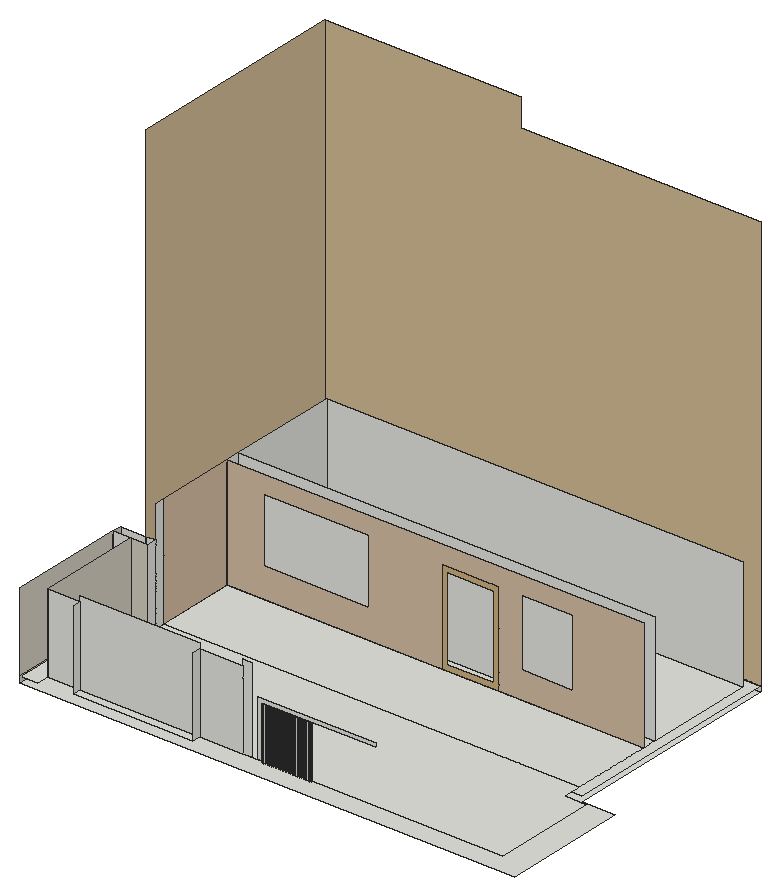
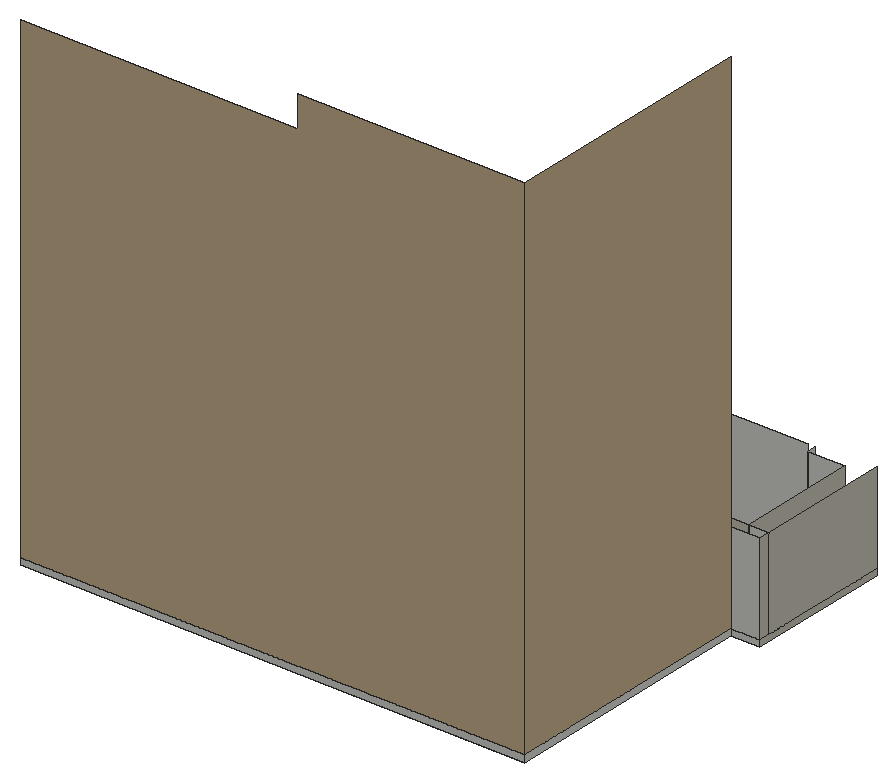
# SketchUp Ruby script. Lengths in inches.
U = 1.inch
M = Sketchup.active_model
def pt(a) = Geom::Point3d.new(a.map { |v| v * U })
def face(e, loops, mat)
  f = e.add_face(loops[0].map { |a| pt(a) })
  loops[1..].each { |l| e.add_face(l.map { |a| pt(a) }).erase! }
  f.material = f.back_material = mat if mat
  f
end
# faces: each face lists its corners as indices into pts; further lists are holes
def faces(e, pts, list, mat = nil) = list.each { |f| face(e, (f[0].is_a?(Array) ? f : [f]).map { |l| l.map { |i| pts[i] } }, mat) }
# xy, xz, yz: faces in a plane at the given z, y or x. An outline is a flat list of corners, or four numbers for a rectangle; further outlines are holes
def ring(l) = l.size == 4 ? [[l[0], l[1]], [l[2], l[1]], [l[2], l[3]], [l[0], l[3]]] : l.each_slice(2).to_a
def flat(e, list, mat, &to3) = list.each { |f| face(e, (f[0].is_a?(Array) ? f : [f]).map { |l| ring(l).map { |u, v| to3.(u, v) } }, mat) }
def xy(e, z, list, mat = nil) = flat(e, list, mat) { |x, y| [x, y, z] }
def xz(e, y, list, mat = nil) = flat(e, list, mat) { |x, z| [x, y, z] }
def yz(e, x, list, mat = nil) = flat(e, list, mat) { |y, z| [x, y, z] }
def lines(e, pts, list) = list.each { |a, b| e.add_line(pt(pts[a]), pt(pts[b])) }
# prism: a flat outline (further loops are holes) pulled along v
def prism(e, loops, v, mat = nil)
  f = face(e, loops, mat); d = Geom::Vector3d.new(v.map { |x| x * U })
  f.pushpull(f.normal.samedirection?(d) ? d.length : -d.length)
end
def box(e, o, s, mat = nil) = prism(e, [[o, [o[0] + s[0], o[1], o[2]], [o[0] + s[0], o[1] + s[1], o[2]], [o[0], o[1] + s[1], o[2]]]], [0, 0, s[2]], mat)
def at(x, y, z, deg = 0) = Geom::Transformation.translation(pt([x, y, z])) * Geom::Transformation.rotation(ORIGIN, Z_AXIS, deg.degrees)
def axes(o, x, y, z) = Geom::Transformation.new([*x, 0, *y, 0, *z, 0, *pt(o).to_a, 1])
def part(name) = M.definitions.add(name)
# library, detail: a bought-in or finely detailed component or shape, given as its bounding box
def library(name, o, s) = part(name).tap { |d| box(d.entities, o, s) }
def detail(e, o, s) = box(e.add_group.entities, o, s)
def put(e, d, t, mat = nil) = e.add_instance(d, t).tap { |i| i.material = mat if mat }
def group(e, t, mat = nil) = e.add_group.tap { |g| g.transformation = t; g.material = mat if mat }.entities
root = M.entities
M.materials.add("[Formica Beige]").color = [211, 187, 149]
M.materials.add("[Formica Graystone]").color = [209, 204, 189]
M.materials.add("[Formica Laminate Light]").color = [213, 189, 164]
M.materials.add("[Wood Floor Light]").color = [204, 176, 127]
xy(root,0,[[0,1.67,0,203.79,40.4375,203.79,40.4375,563.79,742.93,563.79,742.93,203.79,797.12,203.79,797.12,1.67]])
xy(root,9,[[0,1.67,28.1,189.01],[80.35,8.25,273.1875,21.38],[28.1,21.38,762.14,21.38,762.14,189.01,727.17,189.01,727.17,219.56,56.2,219.56,56.2,189.01,28.1,189.01],[0,189.01,56.2,203.79],[40.4375,203.79,40.4375,563.79,742.93,563.79,742.93,203.79,727.17,203.79,727.17,548.03,56.2,548.03,56.2,203.79],
  [56.2,219.56,727.17,348.07],[56.2,348.07,727.17,370.07],[56.2,370.07,727.17,548.03]])
xz(root,17.41,[[370.65,12.5,370.65,102.25,560.77,102.25,560.77,96.37,377.34,96.37,377.34,12.5]])
xz(root,21.38,[[28.1,9,80.35,136.125],[80.35,9,273.1875,145.125],[273.1875,9,342.51,136.125],[342.51,9,357.9375,145.125]])
xz(root,189.01,[[0,9,28.1,136.125]])
xz(root,189.01,[[28.1,9,56.2,136.125]],"[Formica Graystone]")
xz(root,203.79,[[0,0,40.4375,9],[0,9,40.4375,136.125],[40.4375,9,56.2,136.125]])
xz(root,348.07,[[[56.2,9,401.38,9,401.38,160.08,494.76,160.08,494.76,9,727.17,9,727.17,189,56.2,189],[116.08,56.31,284.86,160.63],[530.86,51.82,613.92,160.38]]],"[Formica Laminate Light]")
xz(root,348.07,[[[401.38,9,494.76,160.08],[410.04,17.66,486.1,151.43]]],"[Wood Floor Light]")
xz(root,370.07,[[56.2,9,727.17,189]])
xz(root,548.03,[[56.2,9,727.17,189]])
xz(root,563.79,[[40.4375,0,742.93,9]])
xz(root,563.79,[[40.4375,9,40.4375,723.1875,356.6875,723.1875,356.6875,679.64,742.93,679.64,742.93,9]],"[Formica Beige]")
yz(root,0,[[1.67,0,203.79,9],[1.67,9,189.01,136.125],[189.01,9,203.79,136.125]],"[Formica Graystone]")
yz(root,28.1,[[21.38,9,189.01,136.125]],"[Formica Graystone]")
yz(root,40.4375,[[203.79,0,563.79,9]])
yz(root,40.4375,[[203.79,9,563.79,723.1875]],"[Formica Beige]")
yz(root,56.2,[[189.01,9,203.79,136.125],[203.79,9,219.56,189],[348.07,9,370.07,189],[370.07,9,548.03,189]])
yz(root,56.2,[[219.56,9,348.07,189]],"[Formica Laminate Light]")
yz(root,80.35,[[8.25,9,21.38,136.125]])
yz(root,273.1875,[[8.25,9,21.38,136.125]])
p = [[381.39,13.76,12.5],[381.35,14.08,12.5],[381.35,14.08,96.37],[381.39,13.76,96.37],[383.49,14.08,12.5],[383.45,13.76,12.5],
  [383.45,13.76,96.37],[383.49,14.08,96.37],[385.95,13.76,12.5],[385.91,14.08,12.5],[385.91,14.08,96.37],[385.95,13.76,96.37],
  [389.24,14.08,12.5],[389.2,13.76,12.5],[389.2,13.76,96.37],[389.24,14.08,96.37],[391.7,13.76,12.5],[391.66,14.08,12.5],
  [391.66,14.08,96.37],[391.7,13.76,96.37],[395.74,14.08,12.5],[395.7,13.76,12.5],[395.7,13.76,96.37],[395.74,14.08,96.37],
  [398.2,13.76,12.5],[398.16,14.08,12.5],[398.16,14.08,96.37],[398.2,13.76,96.37],[401.37,14.08,12.5],[401.33,13.76,12.5],
  [401.33,13.76,96.37],[401.37,14.08,96.37],[403.83,13.76,12.5],[403.78,14.08,12.5],[403.78,14.08,96.37],[403.83,13.76,96.37],
  [407.24,14.08,12.5],[407.2,13.76,12.5],[407.2,13.76,96.37],[407.24,14.08,96.37],[409.7,13.76,12.5],[409.66,14.08,12.5],
  [409.66,14.08,96.37],[409.7,13.76,96.37],[412.81,14.08,12.5],[412.76,13.76,12.5],[412.76,13.76,96.37],[412.81,14.08,96.37],
  [415.26,13.76,12.5],[415.22,14.08,12.5],[415.22,14.08,96.37],[415.26,13.76,96.37],[417.68,14.08,12.5],[417.64,13.76,12.5],
  [417.64,13.76,96.37],[417.68,14.08,96.37],[420.14,13.76,12.5],[420.1,14.08,12.5],[420.1,14.08,96.37],[420.14,13.76,96.37],
  [423.43,14.08,12.5],[423.39,13.76,12.5],[423.39,13.76,96.37],[423.43,14.08,96.37],[425.89,13.76,12.5],[425.85,14.08,12.5],
  [425.85,14.08,96.37],[425.89,13.76,96.37],[429.31,14.08,12.5],[429.26,13.76,12.5],[429.26,13.76,96.37],[429.31,14.08,96.37],
  [431.76,13.76,12.5],[431.72,14.08,12.5],[431.72,14.08,96.37],[431.76,13.76,96.37],[434.99,14.08,12.5],[434.95,13.76,12.5],
  [434.95,13.76,96.37],[434.99,14.08,96.37],[437.45,13.76,12.5],[437.41,14.08,12.5],[437.41,14.08,96.37],[437.45,13.76,96.37],
  [441.24,14.08,12.5],[441.2,13.76,12.5],[441.2,13.76,96.37],[441.24,14.08,96.37],[443.7,13.76,12.5],[443.66,14.08,12.5],
  [443.66,14.08,96.37],[443.7,13.76,96.37],[447.24,14.08,12.5],[447.2,13.76,12.5],[447.2,13.76,96.37],[447.24,14.08,96.37],
  [449.7,13.76,12.5],[449.66,14.08,12.5],[449.66,14.08,96.37],[449.7,13.76,96.37],[452.74,14.08,12.5],[452.7,13.76,12.5],
  [452.7,13.76,96.37],[452.74,14.08,96.37],[455.2,13.76,12.5],[455.16,14.08,12.5],[455.16,14.08,96.37],[455.2,13.76,96.37],
  [457.43,14.08,12.5],[457.39,13.76,12.5],[457.39,13.76,96.37],[457.43,14.08,96.37],[379.06,14.38,12.5],[378.94,14.08,12.5],
  [378.94,14.08,96.37],[379.06,14.38,96.37],[381.23,14.38,12.5],[381.23,14.38,96.37],[383.62,14.38,12.5],[383.62,14.38,96.37],
  [385.78,14.38,12.5],[385.78,14.38,96.37],[389.37,14.38,12.5],[389.37,14.38,96.37],[391.53,14.38,12.5],[391.53,14.38,96.37],
  [395.87,14.38,12.5],[395.87,14.38,96.37],[398.03,14.38,12.5],[398.03,14.38,96.37],[401.49,14.38,12.5],[401.49,14.38,96.37],
  [403.66,14.38,12.5],[403.66,14.38,96.37],[407.37,14.38,12.5],[407.37,14.38,96.37],[409.53,14.38,12.5],[409.53,14.38,96.37],
  [412.93,14.38,12.5],[412.93,14.38,96.37],[415.1,14.38,12.5],[415.1,14.38,96.37],[417.81,14.38,12.5],[417.81,14.38,96.37],
  [419.97,14.38,12.5],[419.97,14.38,96.37],[423.56,14.38,12.5],[423.56,14.38,96.37],[425.72,14.38,12.5],[425.72,14.38,96.37],
  [429.43,14.38,12.5],[429.43,14.38,96.37],[431.6,14.38,12.5],[431.6,14.38,96.37],[435.12,14.38,12.5],[435.12,14.38,96.37],
  [437.28,14.38,12.5],[437.28,14.38,96.37],[441.37,14.38,12.5],[441.37,14.38,96.37],[443.53,14.38,12.5],[443.53,14.38,96.37],
  [447.37,14.38,12.5],[447.37,14.38,96.37],[449.53,14.38,12.5],[449.53,14.38,96.37],[452.87,14.38,12.5],[452.87,14.38,96.37],
  [455.03,14.38,12.5],[455.03,14.38,96.37],[457.56,14.38,12.5],[457.56,14.38,96.37],[379.26,14.64,12.5],[379.26,14.64,96.37],
  [381.03,14.64,12.5],[381.03,14.64,96.37],[383.82,14.64,12.5],[383.82,14.64,96.37],[385.59,14.64,12.5],[385.59,14.64,96.37],
  [389.57,14.64,12.5],[389.57,14.64,96.37],[391.34,14.64,12.5],[391.34,14.64,96.37],[396.07,14.64,12.5],[396.07,14.64,96.37],
  [397.84,14.64,12.5],[397.84,14.64,96.37],[401.69,14.64,12.5],[401.69,14.64,96.37],[403.46,14.64,12.5],[403.46,14.64,96.37],
  [407.57,14.64,12.5],[407.57,14.64,96.37],[409.34,14.64,12.5],[409.34,14.64,96.37],[413.13,14.64,12.5],[413.13,14.64,96.37],
  [414.9,14.64,12.5],[414.9,14.64,96.37],[418.01,14.64,12.5],[418.01,14.64,96.37],[419.77,14.64,12.5],[419.77,14.64,96.37],
  [423.76,14.64,12.5],[423.76,14.64,96.37],[425.52,14.64,12.5],[425.52,14.64,96.37],[429.63,14.64,12.5],[429.63,14.64,96.37],
  [431.4,14.64,12.5],[431.4,14.64,96.37],[435.32,14.64,12.5],[435.32,14.64,96.37],[437.09,14.64,12.5],[437.09,14.64,96.37],
  [441.57,14.64,12.5],[441.57,14.64,96.37],[443.34,14.64,12.5],[443.34,14.64,96.37],[447.57,14.64,12.5],[447.57,14.64,96.37],
  [449.34,14.64,12.5],[449.34,14.64,96.37],[453.07,14.64,12.5],[453.07,14.64,96.37],[454.84,14.64,12.5],[454.84,14.64,96.37],
  [457.76,14.64,12.5],[457.76,14.64,96.37],[459.72,14.38,12.5],[459.52,14.64,12.5],[459.52,14.64,96.37],[459.72,14.38,96.37],
  [379.52,14.84,12.5],[379.52,14.84,96.37],[380.77,14.84,12.5],[380.77,14.84,96.37],[384.08,14.84,12.5],[384.08,14.84,96.37],
  [385.33,14.84,12.5],[385.33,14.84,96.37],[389.83,14.84,12.5],[389.83,14.84,96.37],[391.08,14.84,12.5],[391.08,14.84,96.37],
  [396.33,14.84,12.5],[396.33,14.84,96.37],[397.58,14.84,12.5],[397.58,14.84,96.37],[401.95,14.84,12.5],[401.95,14.84,96.37],
  [403.2,14.84,12.5],[403.2,14.84,96.37],[407.83,14.84,12.5],[407.83,14.84,96.37],[409.08,14.84,12.5],[409.08,14.84,96.37],
  [413.39,14.84,12.5],[413.39,14.84,96.37],[414.64,14.84,12.5],[414.64,14.84,96.37],[418.26,14.84,12.5],[418.26,14.84,96.37],
  [419.51,14.84,12.5],[419.51,14.84,96.37],[424.01,14.84,12.5],[424.01,14.84,96.37],[425.26,14.84,12.5],[425.26,14.84,96.37],
  [429.89,14.84,12.5],[429.89,14.84,96.37],[431.14,14.84,12.5],[431.14,14.84,96.37],[435.58,14.84,12.5],[435.58,14.84,96.37],
  [436.83,14.84,12.5],[436.83,14.84,96.37],[441.83,14.84,12.5],[441.83,14.84,96.37],[443.08,14.84,12.5],[443.08,14.84,96.37],
  [447.83,14.84,12.5],[447.83,14.84,96.37],[449.08,14.84,12.5],[449.08,14.84,96.37],[453.33,14.84,12.5],[453.33,14.84,96.37],
  [454.58,14.84,12.5],[454.58,14.84,96.37],[458.01,14.84,12.5],[458.01,14.84,96.37],[459.26,14.84,12.5],[459.26,14.84,96.37],
  [379.82,14.96,12.5],[379.82,14.96,96.37],[380.47,14.96,12.5],[380.47,14.96,96.37],[384.38,14.96,12.5],[384.38,14.96,96.37],
  [385.03,14.96,12.5],[385.03,14.96,96.37],[390.13,14.96,12.5],[390.13,14.96,96.37],[390.78,14.96,12.5],[390.78,14.96,96.37],
  [396.63,14.96,12.5],[396.63,14.96,96.37],[397.28,14.96,12.5],[397.28,14.96,96.37],[402.25,14.96,12.5],[402.25,14.96,96.37],
  [402.9,14.96,12.5],[402.9,14.96,96.37],[408.13,14.96,12.5],[408.13,14.96,96.37],[408.78,14.96,12.5],[408.78,14.96,96.37],
  [413.69,14.96,12.5],[413.69,14.96,96.37],[414.34,14.96,12.5],[414.34,14.96,96.37],[418.57,14.96,12.5],[418.57,14.96,96.37],
  [419.21,14.96,12.5],[419.21,14.96,96.37],[424.32,14.96,12.5],[424.32,14.96,96.37],[424.96,14.96,12.5],[424.96,14.96,96.37],
  [430.19,14.96,12.5],[430.19,14.96,96.37],[430.84,14.96,12.5],[430.84,14.96,96.37],[435.88,14.96,12.5],[435.88,14.96,96.37],
  [436.53,14.96,12.5],[436.53,14.96,96.37],[442.13,14.96,12.5],[442.13,14.96,96.37],[442.78,14.96,12.5],[442.78,14.96,96.37],
  [448.13,14.96,12.5],[448.13,14.96,96.37],[448.78,14.96,12.5],[448.78,14.96,96.37],[453.63,14.96,12.5],[453.63,14.96,96.37],
  [454.28,14.96,12.5],[454.28,14.96,96.37],[458.32,14.96,12.5],[458.32,14.96,96.37],[458.96,14.96,12.5],[458.96,14.96,96.37],
  [380.14,15.01,12.5],[380.14,15.01,96.37],[384.7,15.01,12.5],[384.7,15.01,96.37],[390.45,15.01,12.5],[390.45,15.01,96.37],
  [396.95,15.01,12.5],[396.95,15.01,96.37],[402.58,15.01,12.5],[402.58,15.01,96.37],[408.45,15.01,12.5],[408.45,15.01,96.37],
  [414.01,15.01,12.5],[414.01,15.01,96.37],[418.89,15.01,12.5],[418.89,15.01,96.37],[424.64,15.01,12.5],[424.64,15.01,96.37],
  [430.51,15.01,12.5],[430.51,15.01,96.37],[436.2,15.01,12.5],[436.2,15.01,96.37],[442.45,15.01,12.5],[442.45,15.01,96.37],
  [448.45,15.01,12.5],[448.45,15.01,96.37],[453.95,15.01,12.5],[453.95,15.01,96.37],[458.64,15.01,12.5],[458.64,15.01,96.37]]
faces(root,p,[[0,1,2,3],[4,5,6,7],[8,9,10,11],[12,13,14,15],[16,17,18,19],[20,21,22,23],[24,25,26,27],[28,29,30,31],
  [32,33,34,35],[36,37,38,39],[40,41,42,43],[44,45,46,47],[48,49,50,51],[52,53,54,55],[56,57,58,59],[60,61,62,63],
  [64,65,66,67],[68,69,70,71],[72,73,74,75],[76,77,78,79],[80,81,82,83],[84,85,86,87],[88,89,90,91],[92,93,94,95],
  [96,97,98,99],[100,101,102,103],[104,105,106,107],[108,109,110,111],[112,113,114,115],[1,116,117,2],[118,4,7,119],[9,120,121,10],
  [122,12,15,123],[17,124,125,18],[126,20,23,127],[25,128,129,26],[130,28,31,131],[33,132,133,34],[134,36,39,135],[41,136,137,42],
  [138,44,47,139],[49,140,141,50],[142,52,55,143],[57,144,145,58],[146,60,63,147],[65,148,149,66],[150,68,71,151],[73,152,153,74],
  [154,76,79,155],[81,156,157,82],[158,84,87,159],[89,160,161,90],[162,92,95,163],[97,164,165,98],[166,100,103,167],[105,168,169,106],
  [170,108,111,171],[172,112,115,173],[116,174,175,117],[176,118,119,177],[120,178,179,121],[180,122,123,181],[124,182,183,125],[184,126,127,185],
  [128,186,187,129],[188,130,131,189],[132,190,191,133],[192,134,135,193],[136,194,195,137],[196,138,139,197],[140,198,199,141],[200,142,143,201],
  [144,202,203,145],[204,146,147,205],[148,206,207,149],[208,150,151,209],[152,210,211,153],[212,154,155,213],[156,214,215,157],[216,158,159,217],
  [160,218,219,161],[220,162,163,221],[164,222,223,165],[224,166,167,225],[168,226,227,169],[228,170,171,229],[230,231,232,233],[234,172,173,235],
  [174,236,237,175],[238,176,177,239],[178,240,241,179],[242,180,181,243],[182,244,245,183],[246,184,185,247],[186,248,249,187],[250,188,189,251],
  [190,252,253,191],[254,192,193,255],[194,256,257,195],[258,196,197,259],[198,260,261,199],[262,200,201,263],[202,264,265,203],[266,204,205,267],
  [206,268,269,207],[270,208,209,271],[210,272,273,211],[274,212,213,275],[214,276,277,215],[278,216,217,279],[218,280,281,219],[282,220,221,283],
  [222,284,285,223],[286,224,225,287],[226,288,289,227],[290,228,229,291],[231,292,293,232],[294,234,235,295],[236,296,297,237],[298,238,239,299],
  [240,300,301,241],[302,242,243,303],[244,304,305,245],[306,246,247,307],[248,308,309,249],[310,250,251,311],[252,312,313,253],[314,254,255,315],
  [256,316,317,257],[318,258,259,319],[260,320,321,261],[322,262,263,323],[264,324,325,265],[326,266,267,327],[268,328,329,269],[330,270,271,331],
  [272,332,333,273],[334,274,275,335],[276,336,337,277],[338,278,279,339],[280,340,341,281],[342,282,283,343],[284,344,345,285],[346,286,287,347],
  [288,348,349,289],[350,290,291,351],[292,352,353,293],[354,294,295,355],[296,354,355,297],[356,298,299,357],[300,356,357,301],[358,302,303,359],
  [304,358,359,305],[360,306,307,361],[308,360,361,309],[362,310,311,363],[312,362,363,313],[364,314,315,365],[316,364,365,317],[366,318,319,367],
  [320,366,367,321],[368,322,323,369],[324,368,369,325],[370,326,327,371],[328,370,371,329],[372,330,331,373],[332,372,373,333],[374,334,335,375],
  [336,374,375,337],[376,338,339,377],[340,376,377,341],[378,342,343,379],[344,378,379,345],[380,346,347,381],[348,380,381,349],[382,350,351,383],
  [352,382,383,353]])
